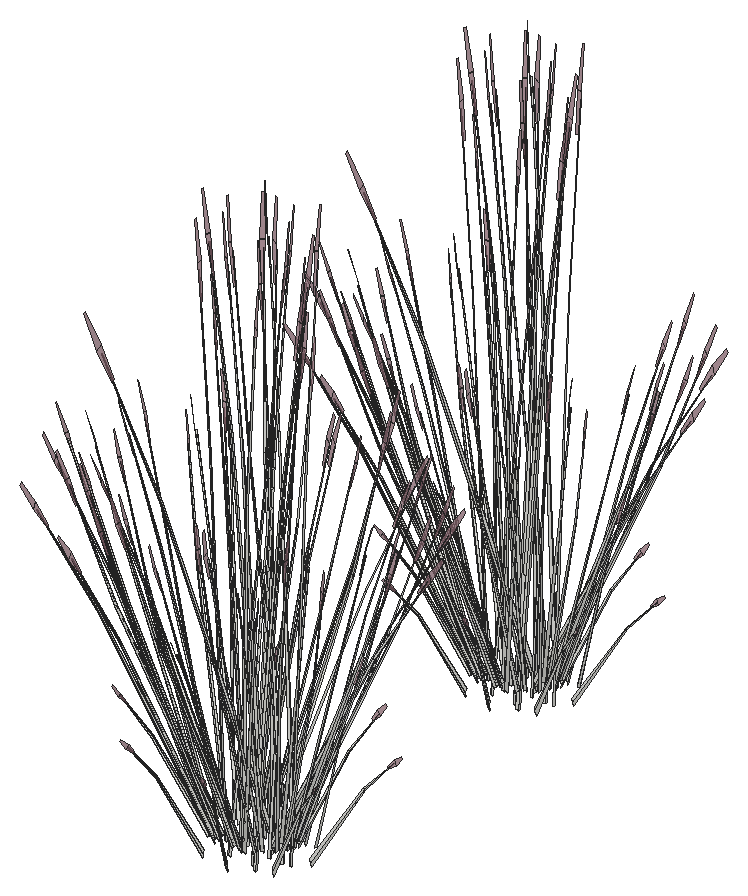
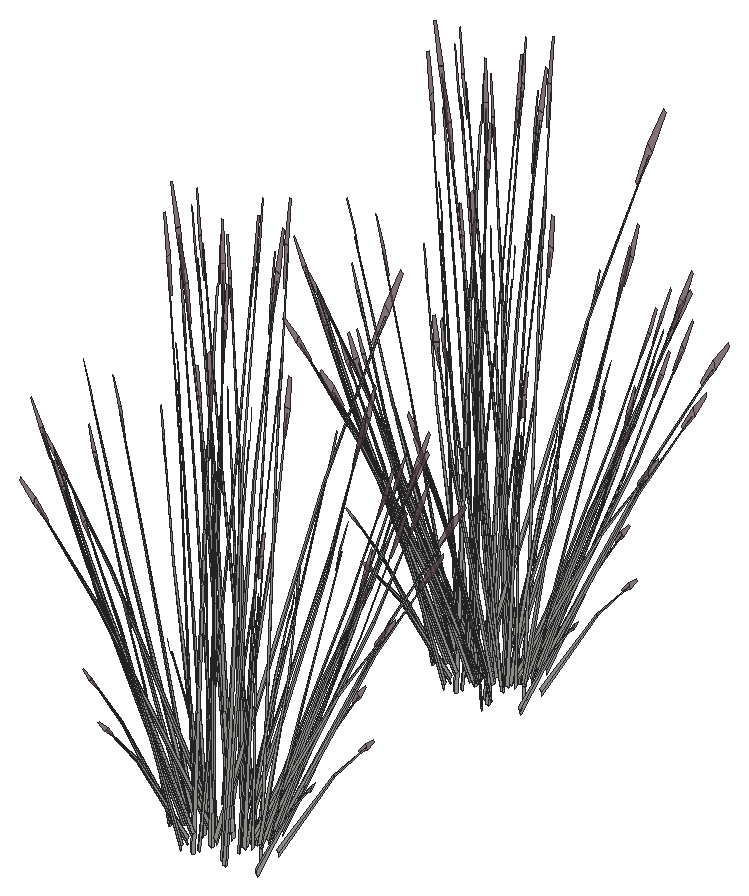
# SketchUp Ruby script. Lengths in inches.
U = 1.inch
M = Sketchup.active_model
def pt(a) = Geom::Point3d.new(a.map { |v| v * U })
def face(e, loops, mat)
  f = e.add_face(loops[0].map { |a| pt(a) })
  loops[1..].each { |l| e.add_face(l.map { |a| pt(a) }).erase! }
  f.material = f.back_material = mat if mat
  f
end
# faces: each face lists its corners as indices into pts; further lists are holes
def faces(e, pts, list, mat = nil) = list.each { |f| face(e, (f[0].is_a?(Array) ? f : [f]).map { |l| l.map { |i| pts[i] } }, mat) }
# xy, xz, yz: faces in a plane at the given z, y or x. An outline is a flat list of corners, or four numbers for a rectangle; further outlines are holes
def ring(l) = l.size == 4 ? [[l[0], l[1]], [l[2], l[1]], [l[2], l[3]], [l[0], l[3]]] : l.each_slice(2).to_a
def flat(e, list, mat, &to3) = list.each { |f| face(e, (f[0].is_a?(Array) ? f : [f]).map { |l| ring(l).map { |u, v| to3.(u, v) } }, mat) }
def xy(e, z, list, mat = nil) = flat(e, list, mat) { |x, y| [x, y, z] }
def xz(e, y, list, mat = nil) = flat(e, list, mat) { |x, z| [x, y, z] }
def yz(e, x, list, mat = nil) = flat(e, list, mat) { |y, z| [x, y, z] }
def lines(e, pts, list) = list.each { |a, b| e.add_line(pt(pts[a]), pt(pts[b])) }
# prism: a flat outline (further loops are holes) pulled along v
def prism(e, loops, v, mat = nil)
  f = face(e, loops, mat); d = Geom::Vector3d.new(v.map { |x| x * U })
  f.pushpull(f.normal.samedirection?(d) ? d.length : -d.length)
end
def box(e, o, s, mat = nil) = prism(e, [[o, [o[0] + s[0], o[1], o[2]], [o[0] + s[0], o[1] + s[1], o[2]], [o[0], o[1] + s[1], o[2]]]], [0, 0, s[2]], mat)
def at(x, y, z, deg = 0) = Geom::Transformation.translation(pt([x, y, z])) * Geom::Transformation.rotation(ORIGIN, Z_AXIS, deg.degrees)
def axes(o, x, y, z) = Geom::Transformation.new([*x, 0, *y, 0, *z, 0, *pt(o).to_a, 1])
def part(name) = M.definitions.add(name)
# library, detail: a bought-in or finely detailed component or shape, given as its bounding box
def library(name, o, s) = part(name).tap { |d| box(d.entities, o, s) }
def detail(e, o, s) = box(e.add_group.entities, o, s)
def put(e, d, t, mat = nil) = e.add_instance(d, t).tap { |i| i.material = mat if mat }
def group(e, t, mat = nil) = e.add_group.tap { |g| g.transformation = t; g.material = mat if mat }.entities
root = M.entities
M.materials.add("LightPink_Translucent").color = [144, 107, 117]
M.materials["LightPink_Translucent"].alpha = 0.75
c1 = part("blade")
p = [[2.15,0.21,22],[0,0.17,0],[0.09,0.45,0],[2.18,0.31,22],[2.29,0.31,22],[0.38,0.45,0],
  [2.48,0.24,33],[2.49,0.24,33],[2.48,0.22,33]]
faces(c1.entities,p,[[0,1,2,3],[4,5,2,3],[6,3,4,7],[8,0,3,6]])
c2 = part("seeds")
p = [[0.3,-0.1,1.38],[-0.01,-0.03,1.59],[-0.01,-0.03,0.03],[0.14,-0.07,-0.07],[0.29,-0.03,3],[0.15,0.01,3.11]]
faces(c2.entities,p,[[0,1,2,3],[1,0,4,5]],"LightPink_Translucent")
c3 = part("blade with seeds")
put(c3.entities,c1,at(0,0,0))
put(c3.entities,c2,axes([2.4,0.25,30.99],[1.5799,-0.05474,1.17369],[-0.12525,1.92788,0.29478],[-0.07173,-0.02425,1.56792]))
put(root,c3,axes([670.27,166.32,513.22],[0.14872,0.18332,1.42242],[-0.6872,0.15433,0.11501],[-0.15531,-0.28779,0.60807]))
put(root,c3,axes([672.1,166.46,514.13],[-0.31051,-0.46426,-0.58968],[0.63919,-0.25873,0.07116],[-0.07261,-0.22432,0.83415]))
put(root,c3,axes([673.39,166.91,514.13],[0.01693,-0.52814,-0.58968],[0.71285,0.03547,0.07116],[0.07523,-0.22375,0.83415]))
put(root,c3,axes([672.16,166.0625,513.76],[0.19614,-0.43908,-0.29394],[0.57222,0.12807,0.37948],[-0.05247,-0.17678,0.72609]))
put(root,c3,axes([672.59,166.64,513.22],[-0.12114,0.19625,1.42242],[-0.50818,-0.40613,0.11501],[0.22925,-0.25313,0.60807]))
put(root,c3,axes([671.87,166.36,513.89],[-0.63954,-0.14313,-0.42412],[0.21921,-0.49074,-0.32852],[-0.05864,-0.19758,0.81151]))
put(root,c3,axes([672.26,165.13,512.3],[0.08346,0.33295,0.95334],[-0.46298,-0.1844,0.70045],[0.04982,-0.17048,0.20998]))
put(root,c3,axes([673.25,166.73,513.89],[-0.46573,-0.38364,-0.42412],[0.49199,-0.33598,-0.32852],[0.07086,-0.19492,0.81151]))
put(root,c3,axes([673.69,166.59,513.76],[0.4402,-0.30062,-0.29394],[0.41671,0.34326,0.37948],[0.0634,-0.1744,0.72609]))
put(root,c3,axes([669.88,165.53,512.3],[0.33937,0.19872,0.95334],[-0.49424,0.11946,0.70045],[-0.10575,-0.15273,0.20998]))
put(root,c3,axes([670.7,166.59,514.13],[-0.55475,-0.27598,-0.58968],[0.39425,-0.48361,0.07116],[-0.20099,-0.16478,0.83415]))
put(root,c3,axes([670.51,166.22,513.76],[-0.10048,-0.4599,-0.29394],[0.5744,-0.12144,0.37948],[-0.15428,-0.13179,0.72609]))
put(root,c3,axes([669.27,166.89,513.22],[0.24166,0.09837,1.42242],[-0.50011,0.41269,0.11501],[-0.3117,-0.18617,0.60807]))
put(root,c3,axes([670.44,166.6,513.89],[-0.64198,0.13573,-0.42412],[-0.1123,-0.514,-0.32852],[-0.17243,-0.1473,0.81151]))
put(root,c3,axes([674.23,167.83,514.13],[0.33983,-0.45051,-0.58968],[0.59551,0.32017,0.07116],[0.20291,-0.16322,0.83415]))
put(root,c3,axes([674.21,167.62,513.89],[-0.16713,-0.52135,-0.42412],[0.63294,-0.0912,-0.32852],[0.18138,-0.14003,0.81151]))
put(root,c3,axes([672.03,169.71,512.76],[0.56221,0.23024,1.25546],[-0.55078,0.49601,0.49647],[-0.2467,-0.29398,1.05249]))
put(root,c3,axes([674.99,166.58,512.3],[-0.2167,0.29065,0.95334],[-0.18626,-0.3905,0.70045],[0.17898,-0.09785,0.20998]))
put(root,c3,axes([674.68,167.67,513.76],[0.56631,-0.0816,-0.29394],[0.14954,0.46647,0.37948],[0.16229,-0.12529,0.72609]))
put(root,c3,axes([669.18,167.03,513.76],[-0.37017,-0.35748,-0.29394],[0.42268,-0.3384,0.37948],[-0.21476,-0.05149,0.72609]))
put(root,c3,axes([669.57,167.27,514.13],[-0.65035,-0.01375,-0.58968],[0.04368,-0.5789,0.07116],[-0.27552,-0.06109,0.83415]))
put(root,c3,axes([669.35,167.39,513.89],[-0.47241,0.37822,-0.42412],[-0.41372,-0.39954,-0.32852],[-0.24002,-0.05755,0.81151]))
put(root,c3,axes([668.29,167.89,512.3],[0.41536,-0.04086,0.95334],[-0.26347,0.35999,0.70045],[-0.20525,-0.054,0.20998]))
put(root,c3,axes([671.22,168.22,512.26],[-0.70648,0.03525,0.37133],[-0.06389,-0.58508,-0.17871],[0.12647,-0.0593,1.19224]))
put(root,c3,axes([669.4,168.65,512.06],[0,0.57097,0.4121],[-0.72788,0,0],[0,-0.13004,1.30728]))
put(root,c3,axes([674.51,168.77,513.89],[0.17625,-0.51936,-0.42412],[0.60429,0.17802,-0.32852],[0.2433,-0.04762,0.81151]))
put(root,c3,axes([668.76,167.79,513.22],[0.26985,-0.01293,1.42242],[-0.17902,0.56047,0.11501],[-0.38456,-0.03467,0.60807]))
put(root,c3,axes([671.06,168.93,512.26],[-0.31565,0.51449,0.37133],[-0.65588,-0.24761,-0.17871],[0,-0.1186,1.19224]))
put(root,c3,axes([673.2,166.96,512.06],[-0.60889,-0.28548,0.4121],[0.36394,-0.51192,0],[0.13868,0.06502,1.30728]))
put(root,c3,axes([674.39,168.96,514.13],[0.57168,-0.25217,-0.58968],[0.3186,0.51908,0.07116],[0.27622,-0.05897,0.83415]))
put(root,c3,axes([670.89,167.22,512.05],[-0.18794,0.56744,0.14643],[-0.68774,-0.16058,0.29122],[0.1188,-0.00276,1.33138]))
put(root,c3,axes([672.07,167.98,512.26],[-0.39083,-0.47924,0.37133],[0.59199,-0.33747,-0.17871],[0.12647,0.0593,1.19224]))
put(root,c3,axes([670.83,170.14,512.05],[0.6991,-0.15154,0.14643],[0.17263,0.56398,0.29122],[-0.06235,-0.08217,1.33138]))
put(root,c3,axes([674.88,169.01,513.76],[0.54068,0.15928,-0.29394],[-0.1577,0.46469,0.37948],[0.21769,-0.04261,0.72609]))
put(root,c3,axes([668.52,168.27,513.76],[-0.54068,-0.15928,-0.29394],[0.1577,-0.46469,0.37948],[-0.21769,0.04261,0.72609]))
put(root,c3,axes([672.97,167.25,512.05],[-0.6991,0.15154,0.14643],[-0.17263,-0.56398,0.29122],[0.06235,0.08217,1.33138]))
put(root,c3,axes([673.41,168.4375,513.22],[-0.26985,0.01293,1.42242],[0.17902,-0.56047,0.11501],[0.38456,0.03467,0.60807]))
put(root,c3,axes([672.91,170.17,512.05],[0.18794,-0.56744,0.14643],[0.68774,0.16058,0.29122],[-0.1188,0.00276,1.33138]))
put(root,c3,axes([670.17,168.19,512.77],[0.18493,-0.0826,1.46963],[0.06377,0.5767,0.11501],[-0.40056,0.07652,0.52526]))
put(root,c3,axes([673.98,168.73,512.05],[-0.51116,-0.4159,0.14643],[0.51512,-0.4034,0.29122],[-0.05645,0.08494,1.33138]))
put(root,c3,axes([676.03,169.11,512.3],[-0.40197,0.09426,0.95334],[0.18921,-0.38956,0.70045],[0.21325,0.02666,0.20998]))
put(root,c3,axes([670.6,170.43,512.06],[0.60889,0.28548,0.4121],[-0.36394,0.51192,0],[-0.13868,-0.06502,1.30728]))
put(root,c3,axes([672.75,168.45,512.26],[0.31565,-0.51449,0.37133],[0.65588,0.24761,-0.17871],[0,0.1186,1.19224]))
put(root,c3,axes([668.89,168.51,513.89],[-0.17625,0.51936,-0.42412],[-0.60429,-0.17802,-0.32852],[-0.2433,0.04762,0.81151]))
put(root,c3,axes([675.33,170.31,513.26],[-0.12452,-0.47997,-0.02898],[0.58854,-0.11034,-0.1314],[0.1229,0.03043,0.43341]))
put(root,c3,axes([674.4,168.74,512.06],[0,-0.57097,0.4121],[0.72788,0,0],[0,0.13004,1.30728]))
put(root,c3,axes([672.58,169.17,512.26],[0.70648,-0.03525,0.37133],[0.06389,0.58508,-0.17871],[-0.12647,0.0593,1.19224]))
put(root,c3,axes([668.875,168.78,513.22],[0.22574,-0.12077,1.42242],[0.19004,0.55807,0.11501],[-0.35439,0.12613,0.60807]))
put(root,c3,axes([673.83,170.01,514.13],[0.65035,0.01375,-0.58968],[-0.04368,0.5789,0.07116],[0.27552,0.06109,0.83415]))
put(root,c3,axes([673.1,170.48,512.06],[0.60889,-0.28548,0.4121],[0.36394,0.51192,0],[-0.13868,0.06502,1.30728]))
put(root,c3,axes([667.7,170.73,512.3],[0.27113,-0.25877,0.95334],[0.10699,0.40966,0.70045],[-0.19594,0.07335,0.20998]))
put(root,c3,axes([674.23,170.25,513.76],[0.37017,0.35748,-0.29394],[-0.42268,0.3384,0.37948],[0.21476,0.05149,0.72609]))
put(root,c3,axes([668.72,169.61,513.76],[-0.56631,0.0816,-0.29394],[-0.14954,-0.46647,0.37948],[-0.16229,0.12529,0.72609]))
put(root,c3,axes([672.9,169.34,513.22],[-0.24166,-0.09837,1.42242],[0.50011,-0.41269,0.11501],[0.3117,0.18617,0.60807]))
put(root,c3,axes([673.79,170.46,512.3],[-0.36631,-0.16417,0.95334],[0.47299,-0.16681,0.70045],[0.12758,0.1413,0.20998]))
put(root,c3,axes([669.7,169.15,513.22],[0.1625,-0.17544,1.42242],[0.41029,0.47354,0.11501],[-0.28141,0.21565,0.60807]))
put(root,c3,axes([669.1875,169.67,513.89],[0.16713,0.52135,-0.42412],[-0.63294,0.0912,-0.32852],[-0.18138,0.14003,0.81151]))
put(root,c3,axes([672.9,168.61,512.36],[-0.01777,-0.53759,1.17256],[0.80434,0.13935,0.49647],[-0.19024,0.29416,1.1068]))
put(root,c3,axes([672.96,170.68,513.89],[0.64198,-0.13573,-0.42412],[0.1123,0.514,-0.32852],[0.17243,0.1473,0.81151]))
put(root,c3,axes([673.85,171.2,512.21],[-0.4172,-0.01791,0.872],[0.27552,-0.38032,0.48145],[0.16481,0.13512,0.68401]))
put(root,c3,axes([669.58,169.58,513.22],[0.12114,-0.19625,1.42242],[0.50818,0.40613,0.11501],[-0.22925,0.25313,0.60807]))
put(root,c3,axes([669.72,170.69,513.76],[-0.4402,0.30062,-0.29394],[-0.41671,-0.34326,0.37948],[-0.0634,0.1744,0.72609]))
put(root,c3,axes([670,171.86,512.3],[-0.01684,-0.3395,0.95334],[0.42072,0.24214,0.70045],[-0.08274,0.16182,0.20998]))
put(root,c3,axes([670.16,170.55,514.15],[0.46573,0.38364,-0.47077],[-0.49199,0.33598,-0.36465],[-0.07086,0.19492,0.90078]))
put(root,c3,axes([671.54,170.92,513.89],[0.63954,0.14313,-0.42412],[-0.21921,0.49074,-0.32852],[0.05864,0.19758,0.81151]))
put(root,c3,axes([671.9,169.91,513.22],[-0.14872,-0.18332,1.42242],[0.6872,-0.15433,0.11501],[0.15531,0.28779,0.60807]))
put(root,c3,axes([671.25,171.22,513.76],[-0.19614,0.43908,-0.29394],[-0.57222,-0.12807,0.37948],[0.05247,0.17678,0.72609]))
put(root,c3,axes([670.01,170.375,514.43],[-0.01693,0.52814,-0.65454],[-0.71285,-0.03547,0.07899],[-0.07523,0.22375,0.92591]))
put(root,c3,axes([670.6875,170,513.22],[-0.01592,-0.21915,1.42242],[0.69015,0.14538,0.11501],[-0.04269,0.3123,0.60807]))
put(root,c3,axes([671.3,170.83,514.13],[0.31051,0.46426,-0.58968],[-0.63919,0.25873,0.07116],[0.07261,0.22432,0.83415]))
put(root,c3,axes([669.77,171.12,512.79],[0.01429,-0.29475,1.28107],[0.64291,0.15569,0.17703],[-0.0557,0.31414,0.60492]))
put(root,c3,axes([670.27,193.78,513.22],[0.14872,0.18332,1.42242],[-0.6872,0.15433,0.11501],[-0.15531,-0.28779,0.60807]))
put(root,c3,axes([672.1,193.91,514.13],[-0.31051,-0.46426,-0.58968],[0.63919,-0.25873,0.07116],[-0.07261,-0.22432,0.83415]))
put(root,c3,axes([673.39,194.37,514.13],[0.01693,-0.52814,-0.58968],[0.71285,0.03547,0.07116],[0.07523,-0.22375,0.83415]))
put(root,c3,axes([672.16,193.52,513.76],[0.19614,-0.43908,-0.29394],[0.57222,0.12807,0.37948],[-0.05247,-0.17678,0.72609]))
put(root,c3,axes([672.59,194.1,513.22],[-0.12114,0.19625,1.42242],[-0.50818,-0.40613,0.11501],[0.22925,-0.25313,0.60807]))
put(root,c3,axes([671.87,193.82,513.89],[-0.63954,-0.14313,-0.42412],[0.21921,-0.49074,-0.32852],[-0.05864,-0.19758,0.81151]))
put(root,c3,axes([672.26,192.59,512.3],[0.08346,0.33295,0.95334],[-0.46298,-0.1844,0.70045],[0.04982,-0.17048,0.20998]))
put(root,c3,axes([673.25,194.19,513.89],[-0.46573,-0.38364,-0.42412],[0.49199,-0.33598,-0.32852],[0.07086,-0.19492,0.81151]))
put(root,c3,axes([673.69,194.05,513.76],[0.4402,-0.30062,-0.29394],[0.41671,0.34326,0.37948],[0.0634,-0.1744,0.72609]))
put(root,c3,axes([669.88,192.99,512.3],[0.33937,0.19872,0.95334],[-0.49424,0.11946,0.70045],[-0.10575,-0.15273,0.20998]))
put(root,c3,axes([670.7,194.04,514.13],[-0.55475,-0.27598,-0.58968],[0.39425,-0.48361,0.07116],[-0.20099,-0.16478,0.83415]))
put(root,c3,axes([670.51,193.68,513.76],[-0.10048,-0.4599,-0.29394],[0.5744,-0.12144,0.37948],[-0.15428,-0.13179,0.72609]))
put(root,c3,axes([669.27,194.35,513.22],[0.24166,0.09837,1.42242],[-0.50011,0.41269,0.11501],[-0.3117,-0.18617,0.60807]))
put(root,c3,axes([670.44,194.06,513.89],[-0.64198,0.13573,-0.42412],[-0.1123,-0.514,-0.32852],[-0.17243,-0.1473,0.81151]))
put(root,c3,axes([674.23,195.28,514.13],[0.33983,-0.45051,-0.58968],[0.59551,0.32017,0.07116],[0.20291,-0.16322,0.83415]))
put(root,c3,axes([674.21,195.07,513.89],[-0.16713,-0.52135,-0.42412],[0.63294,-0.0912,-0.32852],[0.18138,-0.14003,0.81151]))
put(root,c3,axes([672.03,197.17,512.76],[0.56221,0.23024,1.25546],[-0.55078,0.49601,0.49647],[-0.2467,-0.29398,1.05249]))
put(root,c3,axes([674.99,194.04,512.3],[-0.2167,0.29065,0.95334],[-0.18626,-0.3905,0.70045],[0.17898,-0.09785,0.20998]))
put(root,c3,axes([674.68,195.13,513.76],[0.56631,-0.0816,-0.29394],[0.14954,0.46647,0.37948],[0.16229,-0.12529,0.72609]))
put(root,c3,axes([669.18,194.49,513.76],[-0.37017,-0.35748,-0.29394],[0.42268,-0.3384,0.37948],[-0.21476,-0.05149,0.72609]))
put(root,c3,axes([669.57,194.73,514.13],[-0.65035,-0.01375,-0.58968],[0.04368,-0.5789,0.07116],[-0.27552,-0.06109,0.83415]))
put(root,c3,axes([669.35,194.84,513.89],[-0.47241,0.37822,-0.42412],[-0.41372,-0.39954,-0.32852],[-0.24002,-0.05755,0.81151]))
put(root,c3,axes([668.29,195.34,512.3],[0.41536,-0.04086,0.95334],[-0.26347,0.35999,0.70045],[-0.20525,-0.054,0.20998]))
put(root,c3,axes([671.22,195.68,512.26],[-0.70648,0.03525,0.37133],[-0.06389,-0.58508,-0.17871],[0.12647,-0.0593,1.19224]))
put(root,c3,axes([669.4,196.1,512.06],[0,0.57097,0.4121],[-0.72788,0,0],[0,-0.13004,1.30728]))
put(root,c3,axes([674.51,196.23,513.89],[0.17625,-0.51936,-0.42412],[0.60429,0.17802,-0.32852],[0.2433,-0.04762,0.81151]))
put(root,c3,axes([668.76,195.25,513.22],[0.26985,-0.01293,1.42242],[-0.17902,0.56047,0.11501],[-0.38456,-0.03467,0.60807]))
put(root,c3,axes([671.06,196.39,512.26],[-0.31565,0.51449,0.37133],[-0.65588,-0.24761,-0.17871],[0,-0.1186,1.19224]))
put(root,c3,axes([673.2,194.42,512.06],[-0.60889,-0.28548,0.4121],[0.36394,-0.51192,0],[0.13868,0.06502,1.30728]))
put(root,c3,axes([674.39,196.42,514.13],[0.57168,-0.25217,-0.58968],[0.3186,0.51908,0.07116],[0.27622,-0.05897,0.83415]))
put(root,c3,axes([670.89,194.67,512.05],[-0.18794,0.56744,0.14643],[-0.68774,-0.16058,0.29122],[0.1188,-0.00276,1.33138]))
put(root,c3,axes([672.07,195.4375,512.26],[-0.39083,-0.47924,0.37133],[0.59199,-0.33747,-0.17871],[0.12647,0.0593,1.19224]))
put(root,c3,axes([670.83,197.6,512.05],[0.6991,-0.15154,0.14643],[0.17263,0.56398,0.29122],[-0.06235,-0.08217,1.33138]))
put(root,c3,axes([674.88,196.47,513.76],[0.54068,0.15928,-0.29394],[-0.1577,0.46469,0.37948],[0.21769,-0.04261,0.72609]))
put(root,c3,axes([668.52,195.73,513.76],[-0.54068,-0.15928,-0.29394],[0.1577,-0.46469,0.37948],[-0.21769,0.04261,0.72609]))
put(root,c3,axes([672.97,194.7,512.05],[-0.6991,0.15154,0.14643],[-0.17263,-0.56398,0.29122],[0.06235,0.08217,1.33138]))
put(root,c3,axes([673.41,195.89,513.22],[-0.26985,0.01293,1.42242],[0.17902,-0.56047,0.11501],[0.38456,0.03467,0.60807]))
put(root,c3,axes([672.91,197.63,512.05],[0.18794,-0.56744,0.14643],[0.68774,0.16058,0.29122],[-0.1188,0.00276,1.33138]))
put(root,c3,axes([670.17,195.65,512.77],[0.18493,-0.0826,1.46963],[0.06377,0.5767,0.11501],[-0.40056,0.07652,0.52526]))
put(root,c3,axes([673.98,196.18,512.05],[-0.51116,-0.4159,0.14643],[0.51512,-0.4034,0.29122],[-0.05645,0.08494,1.33138]))
put(root,c3,axes([676.03,196.5625,512.3],[-0.40197,0.09426,0.95334],[0.18921,-0.38956,0.70045],[0.21325,0.02666,0.20998]))
put(root,c3,axes([670.6,197.89,512.06],[0.60889,0.28548,0.4121],[-0.36394,0.51192,0],[-0.13868,-0.06502,1.30728]))
put(root,c3,axes([672.75,195.91,512.26],[0.31565,-0.51449,0.37133],[0.65588,0.24761,-0.17871],[0,0.1186,1.19224]))
put(root,c3,axes([668.89,195.97,513.89],[-0.17625,0.51936,-0.42412],[-0.60429,-0.17802,-0.32852],[-0.2433,0.04762,0.81151]))
put(root,c3,axes([675.33,197.76,513.26],[-0.12452,-0.47997,-0.02898],[0.58854,-0.11034,-0.1314],[0.1229,0.03043,0.43341]))
put(root,c3,axes([674.4,196.2,512.06],[0,-0.57097,0.4121],[0.72788,0,0],[0,0.13004,1.30728]))
put(root,c3,axes([672.58,196.625,512.26],[0.70648,-0.03525,0.37133],[0.06389,0.58508,-0.17871],[-0.12647,0.0593,1.19224]))
put(root,c3,axes([668.875,196.23,513.22],[0.22574,-0.12077,1.42242],[0.19004,0.55807,0.11501],[-0.35439,0.12613,0.60807]))
put(root,c3,axes([673.83,197.47,514.13],[0.65035,0.01375,-0.58968],[-0.04368,0.5789,0.07116],[0.27552,0.06109,0.83415]))
put(root,c3,axes([673.1,197.93,512.06],[0.60889,-0.28548,0.4121],[0.36394,0.51192,0],[-0.13868,0.06502,1.30728]))
put(root,c3,axes([667.7,198.1875,512.3],[0.27113,-0.25877,0.95334],[0.10699,0.40966,0.70045],[-0.19594,0.07335,0.20998]))
put(root,c3,axes([674.23,197.71,513.76],[0.37017,0.35748,-0.29394],[-0.42268,0.3384,0.37948],[0.21476,0.05149,0.72609]))
put(root,c3,axes([668.72,197.07,513.76],[-0.56631,0.0816,-0.29394],[-0.14954,-0.46647,0.37948],[-0.16229,0.12529,0.72609]))
put(root,c3,axes([672.9,196.79,513.22],[-0.24166,-0.09837,1.42242],[0.50011,-0.41269,0.11501],[0.3117,0.18617,0.60807]))
put(root,c3,axes([673.79,197.91,512.3],[-0.36631,-0.16417,0.95334],[0.47299,-0.16681,0.70045],[0.12758,0.1413,0.20998]))
put(root,c3,axes([669.7,196.61,513.22],[0.1625,-0.17544,1.42242],[0.41029,0.47354,0.11501],[-0.28141,0.21565,0.60807]))
put(root,c3,axes([669.1875,197.125,513.89],[0.16713,0.52135,-0.42412],[-0.63294,0.0912,-0.32852],[-0.18138,0.14003,0.81151]))
put(root,c3,axes([672.9,196.07,512.36],[-0.01777,-0.53759,1.17256],[0.80434,0.13935,0.49647],[-0.19024,0.29416,1.1068]))
put(root,c3,axes([672.96,198.14,513.89],[0.64198,-0.13573,-0.42412],[0.1123,0.514,-0.32852],[0.17243,0.1473,0.81151]))
put(root,c3,axes([673.85,198.66,512.21],[-0.4172,-0.01791,0.872],[0.27552,-0.38032,0.48145],[0.16481,0.13512,0.68401]))
put(root,c3,axes([669.58,197.04,513.22],[0.12114,-0.19625,1.42242],[0.50818,0.40613,0.11501],[-0.22925,0.25313,0.60807]))
